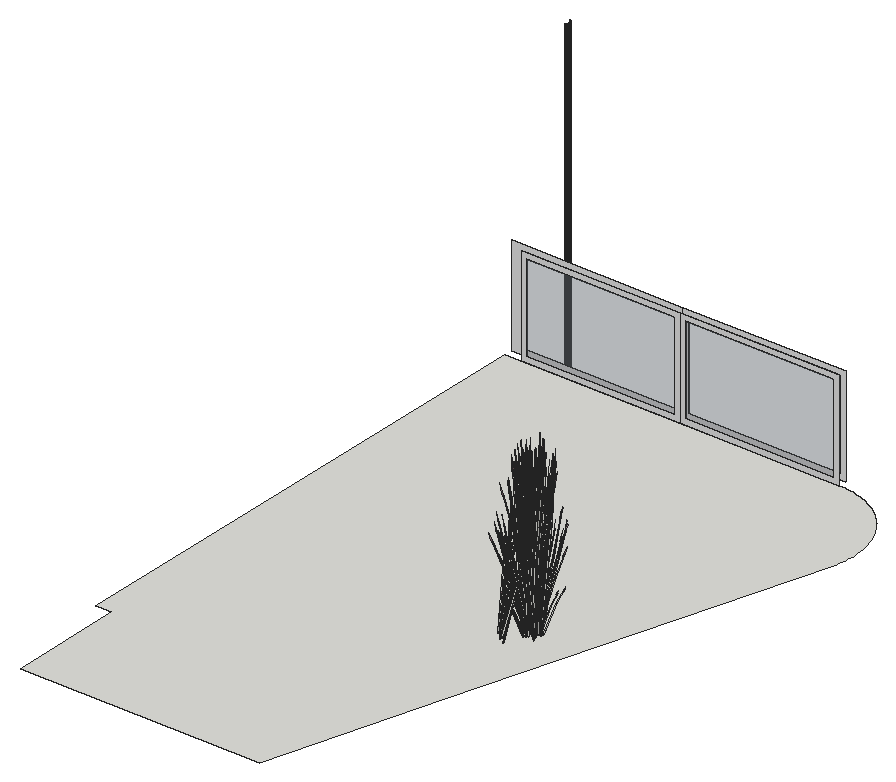
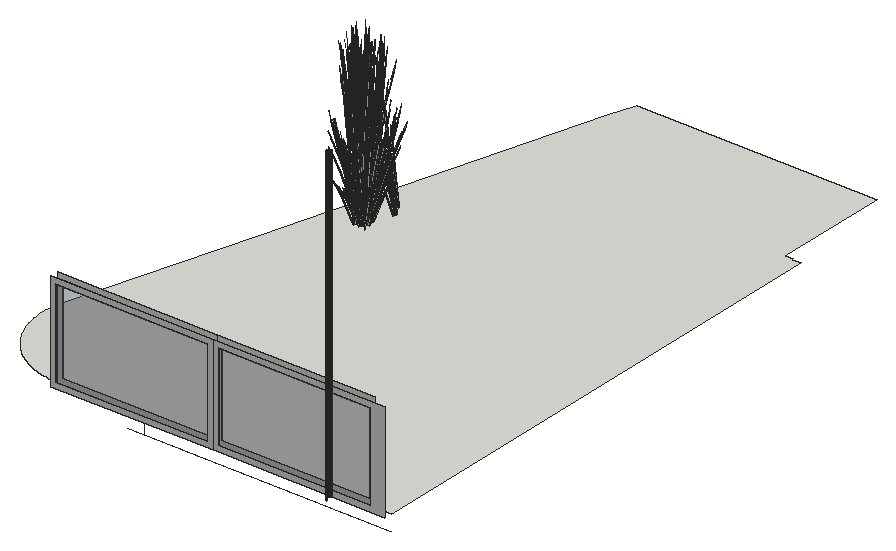
# SketchUp Ruby script. Lengths in inches.
U = 1.inch
M = Sketchup.active_model
def pt(a) = Geom::Point3d.new(a.map { |v| v * U })
def face(e, loops, mat)
  f = e.add_face(loops[0].map { |a| pt(a) })
  loops[1..].each { |l| e.add_face(l.map { |a| pt(a) }).erase! }
  f.material = f.back_material = mat if mat
  f
end
# faces: each face lists its corners as indices into pts; further lists are holes
def faces(e, pts, list, mat = nil) = list.each { |f| face(e, (f[0].is_a?(Array) ? f : [f]).map { |l| l.map { |i| pts[i] } }, mat) }
# xy, xz, yz: faces in a plane at the given z, y or x. An outline is a flat list of corners, or four numbers for a rectangle; further outlines are holes
def ring(l) = l.size == 4 ? [[l[0], l[1]], [l[2], l[1]], [l[2], l[3]], [l[0], l[3]]] : l.each_slice(2).to_a
def flat(e, list, mat, &to3) = list.each { |f| face(e, (f[0].is_a?(Array) ? f : [f]).map { |l| ring(l).map { |u, v| to3.(u, v) } }, mat) }
def xy(e, z, list, mat = nil) = flat(e, list, mat) { |x, y| [x, y, z] }
def xz(e, y, list, mat = nil) = flat(e, list, mat) { |x, z| [x, y, z] }
def yz(e, x, list, mat = nil) = flat(e, list, mat) { |y, z| [x, y, z] }
def lines(e, pts, list) = list.each { |a, b| e.add_line(pt(pts[a]), pt(pts[b])) }
# prism: a flat outline (further loops are holes) pulled along v
def prism(e, loops, v, mat = nil)
  f = face(e, loops, mat); d = Geom::Vector3d.new(v.map { |x| x * U })
  f.pushpull(f.normal.samedirection?(d) ? d.length : -d.length)
end
def box(e, o, s, mat = nil) = prism(e, [[o, [o[0] + s[0], o[1], o[2]], [o[0] + s[0], o[1] + s[1], o[2]], [o[0], o[1] + s[1], o[2]]]], [0, 0, s[2]], mat)
def at(x, y, z, deg = 0) = Geom::Transformation.translation(pt([x, y, z])) * Geom::Transformation.rotation(ORIGIN, Z_AXIS, deg.degrees)
def axes(o, x, y, z) = Geom::Transformation.new([*x, 0, *y, 0, *z, 0, *pt(o).to_a, 1])
def part(name) = M.definitions.add(name)
# library, detail: a bought-in or finely detailed component or shape, given as its bounding box
def library(name, o, s) = part(name).tap { |d| box(d.entities, o, s) }
def detail(e, o, s) = box(e.add_group.entities, o, s)
def put(e, d, t, mat = nil) = e.add_instance(d, t).tap { |i| i.material = mat if mat }
def group(e, t, mat = nil) = e.add_group.tap { |g| g.transformation = t; g.material = mat if mat }.entities
root = M.entities
M.materials.add("Glass_Basic_01").color = [105, 113, 122]
M.materials["Glass_Basic_01"].alpha = 0.25
M.materials.add("LightPink_Translucent").color = [144, 107, 117]
M.materials["LightPink_Translucent"].alpha = 0.75
M.materials.add("M01_Silver_Fog").color = [224, 224, 224]
c1 = part("blade")
p = [[2.15,0.21,22],[0,0.17,0],[0.09,0.45,0],[2.18,0.31,22],[2.29,0.31,22],[0.38,0.45,0],
  [2.48,0.24,33],[2.49,0.24,33],[2.48,0.22,33]]
faces(c1.entities,p,[[0,1,2,3],[4,5,2,3],[6,3,4,7],[8,0,3,6]])
c2 = part("seeds")
p = [[0.3,-0.1,1.38],[-0.01,-0.03,1.59],[-0.01,-0.03,0.03],[0.14,-0.07,-0.07],[0.29,-0.03,3],[0.15,0.01,3.11]]
faces(c2.entities,p,[[0,1,2,3],[1,0,4,5]],"LightPink_Translucent")
c3 = part("blade with seeds")
put(c3.entities,c1,at(0,0,0))
put(c3.entities,c2,axes([2.4,0.25,30.99],[1.5799,-0.05474,1.17369],[-0.12525,1.92788,0.29478],[-0.07173,-0.02425,1.56792]))
xy(root,522,[[216,246,303.26,246,306,255.36,321.22,307.35,340.07,371.78,359.17,437.01,359.4,437.91,359.63,439,359.83,440.1,359.98,441.21,360.09,442.32,360.16,443.43,360.1875,444.55,360.17,445.67,360.11,446.78,360.01,447.89,359.87,449,359.68,450.1,359.45,451.2,359.18,452.28,358.875,453.35,358.52,454.41,358.13,455.46,357.7,456.49,357.23,457.5,356.73,458.5,356.18,459.47,355.6,460.43,354.98,461.36,354.33,462.26,353.64,463.14,352.92,464,352.17,464.83,351.39,465.62,350.58,466.39,349.74,467.125,348.87,467.83,347.97,468.5,347.05,469.13,346.11,469.73,345.15,470.29,344.16,470.82,343.16,471.3,342.13,471.75,341.09,472.16,340.04,472.53,338.97,472.86,337.89,473.15,336.8,473.4,335.71,473.6,334.6,473.77,333.49,473.89,332.38,473.97,331.45,474,210,474,210,288,213,288,213,287.79,216,287.79]])
xz(root,474,[[218,524,271.49,556],[275.49,524,329.45,556]],"Glass_Basic_01")
xz(root,474,[[[216,522,273.49,558],[218,524,271.49,556]],[[273.49,522,331.45,558],[275.49,524,329.45,556]]],"M01_Silver_Fog")
xz(root,477,[[215,524,270.25,556],[274.25,524,329.5,556]],"Glass_Basic_01")
xz(root,477,[[[210,522,272.25,558],[215,524,270.25,556]],[[272.25,522,331.5,558],[274.25,524,329.5,556]]],"M01_Silver_Fog")
yz(root,229.87,[[478.39,522,478.47,635.24]],"M01_Silver_Fog")
p = [[229.03,477.14,522],[229.11,477.18,522],[229.11,477.18,635.24],[229.03,477.14,635.24],[229.18,477.22,522],[229.18,477.22,635.24],
  [229.26,477.27,522],[229.26,477.27,635.24],[229.33,477.32,522],[229.33,477.32,635.24],[229.4,477.38,522],[229.4,477.38,635.24],
  [229.46,477.4375,522],[229.46,477.4375,635.24],[229.52,477.5,522],[229.52,477.5,635.24],[229.58,477.57,522],[229.58,477.57,635.24],
  [229.63,477.64,522],[229.63,477.64,635.24],[229.67,477.72,522],[229.67,477.72,635.24],[229.72,477.79,522],[229.72,477.79,635.24],
  [229.75,477.875,522],[229.75,477.875,635.24],[229.79,477.96,522],[229.79,477.96,635.24],[229.8125,478.04,522],[229.8125,478.04,635.24],
  [229.83,478.125,522],[229.83,478.125,635.24],[229.85,478.21,522],[229.85,478.21,635.24],[229.86,478.3,522],[229.86,478.3,635.24],
  [229.87,478.39,522],[229.87,478.39,635.24],[229.87,478.47,522],[229.86,478.5625,522],[229.86,478.5625,635.24],[229.87,478.47,635.24],
  [229.85,478.65,522],[229.83,478.74,522],[229.83,478.74,635.24],[229.85,478.65,635.24],[229.81,478.82,522],[229.81,478.82,635.24],
  [229.78,478.9,522],[229.78,478.9,635.24],[229.75,478.99,522],[229.75,478.99,635.24],[229.71,479.07,522],[229.71,479.07,635.24],
  [229.67,479.14,522],[229.62,479.22,522],[229.62,479.22,635.24],[229.67,479.14,635.24],[229.57,479.29,522],[229.57,479.29,635.24],
  [229.51,479.35,522],[229.51,479.35,635.24],[229.45,479.42,522],[229.39,479.48,522],[229.39,479.48,635.24],[229.45,479.42,635.24],
  [229.32,479.53,522],[229.25,479.59,522],[229.25,479.59,635.24],[229.32,479.53,635.24],[229.18,479.63,522],[229.1,479.68,522],
  [229.1,479.68,635.24],[229.18,479.63,635.24],[229.02,479.71,522],[229.02,479.71,635.24],[300,474,516],[300,474,522],
  [210,474,516],[306,474,516]]
faces(root,p,[[0,1,2,3],[1,4,5,2],[4,6,7,5],[6,8,9,7],[8,10,11,9],[10,12,13,11],[12,14,15,13],[14,16,17,15],
  [16,18,19,17],[18,20,21,19],[20,22,23,21],[22,24,25,23],[24,26,27,25],[26,28,29,27],[28,30,31,29],[30,32,33,31],
  [32,34,35,33],[34,36,37,35],[38,39,40,41],[42,43,44,45],[39,42,45,40],[43,46,47,44],[46,48,49,47],[48,50,51,49],
  [50,52,53,51],[54,55,56,57],[52,54,57,53],[55,58,59,56],[58,60,61,59],[62,63,64,65],[60,62,65,61],[66,67,68,69],
  [63,66,69,64],[70,71,72,73],[67,70,73,68],[71,74,75,72]],"M01_Silver_Fog")
lines(root,p,[[76,77],[76,78],[76,79]])
put(root,c3,axes([317.24,349.05,525.875],[0.20841,-0.0122,1.71376],[-0.13825,0.52864,0.13857],[-0.297,-0.0327,0.73262]))
put(root,c3,axes([314.15,341.54,524.59],[0.15856,-0.08496,1.43002],[0.39147,0.25616,-0.30754],[-0.11652,0.22165,0.61141]))
put(root,c3,axes([317.33,349.98,525.875],[0.17434,-0.11391,1.71376],[0.14677,0.52637,0.13857],[-0.27369,0.11897,0.73262]))
put(root,c3,axes([316.79,350.875,524.59],[0.17462,0.04421,1.43002],[0.11254,0.45156,-0.30754],[-0.23719,0.08453,0.61141]))
put(root,c3,axes([314.3125,340.72,526.53],[-0.33997,0.28354,-0.35414],[-0.32182,-0.32376,0.4572],[-0.04897,0.1645,0.87481]))
put(root,c3,axes([318.33,349.43,525.34],[0.14282,-0.0779,1.77064],[0.04925,0.54394,0.13857],[-0.30935,0.07218,0.63284]))
put(root,c3,axes([317.87,348.56,526.98],[-0.50227,-0.01297,-0.71045],[0.03373,-0.54602,0.08574],[-0.21278,-0.05762,1.00501]))
put(root,c3,axes([314.54,340.42,527.34],[-0.01307,0.49815,-0.7886],[-0.55054,-0.03346,0.09517],[-0.0581,0.21104,1.11556]))
put(root,c3,axes([317.46,348.69,524.59],[0.0981,0.14994,1.43002],[-0.22605,0.40756,-0.30754],[-0.23211,-0.09741,0.61141]))
put(root,c3,axes([314.53,341.82,524.77],[-0.013,-0.32022,1.1486],[0.32493,0.22839,0.84392],[-0.0639,0.15263,0.25299]))
put(root,c3,axes([317.0625,349.5,526.53],[-0.41757,-0.15024,-0.35414],[0.12179,-0.4383,0.4572],[-0.16812,0.04019,0.87481]))
put(root,c3,axes([317.64,348.2,525.875],[0.18664,0.09279,1.71376],[-0.38624,0.38925,0.13857],[-0.24072,-0.1756,0.73262]))
put(root,c3,axes([317.35,349.73,526.68],[-0.13612,0.48987,-0.51099],[-0.46669,-0.16791,-0.3958],[-0.1879,0.04492,0.97773]))
put(root,c3,axes([314.35,341.12,525.36],[0.01104,-0.27801,1.54345],[0.49652,0.14685,0.21329],[-0.04302,0.2963,0.72882]))
put(root,c3,axes([317.7,348.67,526.68],[-0.36484,0.35674,-0.51099],[-0.31952,-0.37685,-0.3958],[-0.18537,-0.05428,0.97773]))
put(root,c3,axes([317.11,349.7,523.49],[0.01274,0.08487,1.76342],[-0.25688,0.44323,-0.26939],[-0.18246,-0.02234,0.30037]))
put(root,c3,axes([316.42,351.82,524.77],[0.2094,-0.24408,1.1486],[0.08263,0.38639,0.84392],[-0.15132,0.06919,0.25299]))
put(root,c3,axes([314.65,340.59,527],[0.35968,0.36185,-0.5672],[-0.37996,0.3169,-0.43934],[-0.05473,0.18385,1.08528]))
put(root,c3,axes([317.57,348.33,526.53],[-0.28589,-0.33718,-0.35414],[0.32644,-0.31919,0.4572],[-0.16586,-0.04856,0.87481]))
put(root,c3,axes([317.97,350.33,525.875],[0.1255,-0.16547,1.71376],[0.31687,0.44665,0.13857],[-0.21734,0.2034,0.73262]))
put(root,c3,axes([317.21,350.77,526.53],[-0.43736,0.07697,-0.35414],[-0.11549,-0.43998,0.4572],[-0.12533,0.11818,0.87481]))
put(root,c3,axes([316.98,352.07,523.49],[0.0674,0.0538,1.76342],[0.11428,0.49852,-0.26939],[-0.14937,0.10631,0.30037]))
put(root,c3,axes([314.26,341.13,524.82],[0.45645,-0.09537,0.06507],[0.10494,0.38421,-0.86304],[-0.02894,0.19449,0.7736]))
put(root,c3,axes([316.88,349.14,524.77],[0.32078,-0.03854,1.1486],[-0.20348,0.33954,0.84392],[-0.15852,-0.05093,0.25299]))
put(root,c3,axes([315.06,340.07,525.875],[-0.0123,-0.2067,1.71376],[0.53301,0.13712,0.13857],[-0.03297,0.29456,0.73262]))
put(root,c3,axes([317.875,350.74,525.875],[0.09355,-0.18511,1.71376],[0.39247,0.38307,0.13857],[-0.17705,0.23875,0.73262]))
put(root,c3,axes([317.57,350.82,526.68],[0.12908,0.49174,-0.51099],[-0.48882,0.08602,-0.3958],[-0.14008,0.13208,0.97773]))
put(root,c3,axes([318.79,350.47,524.06],[-0.52267,-0.08829,-0.62353],[0.11029,-0.54463,-0.16365],[-0.15598,-0.06599,1.37633]))
put(root,c3,axes([318.74,347.91,526.98],[-0.42844,-0.2603,-0.71045],[0.30448,-0.45614,0.08574],[-0.15523,-0.15542,1.00501]))
put(root,c3,axes([318.54,347.93,526.68],[-0.4958,0.12802,-0.51099],[-0.08673,-0.48481,-0.3958],[-0.13317,-0.13893,0.97773]))
put(root,c3,axes([318.11,351.5,524.02],[-0.47024,-0.26927,-0.49651],[0.28107,-0.48284,0],[-0.1071,-0.06133,1.57504]))
put(root,c3,axes([317.9,347.49,523.49],[-0.04867,0.07094,1.76342],[-0.49185,0.15296,-0.26939],[-0.11882,-0.13915,0.30037]))
put(root,c3,axes([318.39,351.82,524.375],[-0.31414,0.53965,0],[-0.52557,-0.30095,-0.51607],[-0.1197,-0.06854,1.63711]))
put(root,c3,axes([315.38,341.06,523.49],[0.08132,-0.0293,1.76342],[0.48914,0.1613,-0.26939],[0.0143,0.18179,0.30037]))
put(root,c3,axes([315.49,341.22,526.53],[-0.15148,0.41415,-0.35414],[-0.44193,-0.12079,0.4572],[0.04052,0.16674,0.87481]))
put(root,c3,axes([317.82,352.6,524.59],[0.15856,-0.08496,1.43002],[0.39147,0.25616,-0.30754],[-0.11652,0.22165,0.61141]))
put(root,c3,axes([317.6,347.76,524.13],[-0.14494,0.43975,-0.03893],[-0.4461,-0.13527,-0.17649],[-0.06773,-0.07192,0.58215]))
put(root,c3,axes([319.39,350.55,524.67],[-0.5073,0.35754,-0.29095],[-0.33735,-0.5052,-0.50002],[-0.12516,-0.05131,1.59708]))
put(root,c3,axes([318.59,347.57,526.53],[-0.0776,-0.43378,-0.35414],[0.44361,-0.11454,0.4572],[-0.11915,-0.12431,0.87481]))
put(root,c3,axes([317.36,349.77,524.375],[-0.62828,0,0],[0,-0.6019,-0.51607],[0,-0.13709,1.63711]))
put(root,c3,axes([318.24,351.3,524.03],[-0.11803,-0.46926,-0.30978],[0.46876,-0.13325,0.30978],[-0.0945,-0.05411,1.38974]))
put(root,c3,axes([317.98,351.79,526.53],[-0.33997,0.28354,-0.35414],[-0.32182,-0.32376,0.4572],[-0.04897,0.1645,0.87481]))
put(root,c3,axes([319.72,350.9375,524.06],[-0.33843,0.40479,-0.62353],[-0.42041,-0.36705,-0.16365],[-0.13561,0.10098,1.37633]))
put(root,c3,axes([317.84,349.61,524.33],[-0.46736,0.45277,0.30756],[-0.46764,-0.44801,-0.36492],[-0.01632,-0.12858,1.64885]))
put(root,c3,axes([315.54,340.85,526.98],[0.23981,0.43789,-0.71045],[-0.49365,0.24404,0.08574],[0.05608,0.21158,1.00501]))
put(root,c3,axes([319.77,350.86,525.33],[0.4342,0.21716,1.51261],[-0.42537,0.46784,0.59816],[-0.19053,-0.27728,1.26806]))
put(root,c3,axes([318.11,346.92,524.77],[0.2621,0.18744,1.1486],[-0.38171,0.11267,0.84392],[-0.08167,-0.14405,0.25299]))
put(root,c3,axes([319.96,350.71,524.46],[-0.49063,-0.43346,-0.25192],[0.41285,-0.48673,0.5513],[-0.13212,0.05071,1.68216]))
put(root,c3,axes([319.06,350.29,524.21],[-0.30184,-0.45202,-0.44739],[0.45719,-0.31831,0.21531],[-0.09768,-0.05593,1.43643]))
put(root,c3,axes([318.21,351.49,527.34],[-0.01307,0.49815,-0.7886],[-0.55054,-0.03346,0.09517],[-0.0581,0.21104,1.11556]))
put(root,c3,axes([318.2,352.89,524.77],[-0.013,-0.32022,1.1486],[0.32493,0.22839,0.84392],[-0.0639,0.15263,0.25299]))
put(root,c3,axes([319.71,350.62,524.21],[-0.54562,0.03324,-0.44739],[-0.04934,-0.55185,0.21531],[-0.09768,0.05593,1.43643]))
put(root,c3,axes([315.72,340.9375,526.68],[0.49392,0.135,-0.51099],[-0.1693,0.46287,-0.3958],[0.04529,0.18636,0.97773]))
put(root,c3,axes([318.66,351.54,524.48],[0.47024,0.26927,0.49651],[-0.28107,0.48284,0],[-0.1071,-0.06133,1.57504]))
put(root,c3,axes([318.03,352.1875,525.36],[0.01104,-0.27801,1.54345],[0.49652,0.14685,0.21329],[-0.04302,0.2963,0.72882]))
put(root,c3,axes([319.11,350.55,524.4375],[0.13317,-0.63814,-0.23429],[0.63143,0.11124,0.51271],[-0.11033,-0.08813,1.5644]))
put(root,c3,axes([319.34,350.7,524.62],[-0.09693,0.48062,0.1448],[-0.47357,-0.08343,-0.41347],[-0.08619,-0.04935,1.26744]))
put(root,c3,axes([320.28,352.04,524.02],[-0.47024,0.26927,-0.49651],[-0.28107,-0.48284,0],[-0.1071,0.06133,1.57504]))
put(root,c3,axes([317.5,349.36,524.02],[0,-0.53854,-0.49651],[0.56215,0,0],[0,-0.12266,1.57504]))
put(root,c3,axes([317.74,349.86,524.48],[0,0.53854,0.49651],[-0.56215,0,0],[0,-0.12266,1.57504]))
put(root,c3,axes([320.3125,351.9,524.19],[-0.31023,-0.54153,-0.05142],[0.52557,-0.30095,0.51607],[-0.12951,0.05156,1.6363]))
put(root,c3,axes([318.32,351.65,527],[0.35968,0.36185,-0.5672],[-0.37996,0.3169,-0.43934],[-0.05473,0.18385,1.08528]))
put(root,c3,axes([320.17,351.83,524.03],[-0.46876,-0.13325,-0.30978],[0.11803,-0.46926,0.30978],[-0.0945,0.05411,1.38974]))
put(root,c3,axes([318.97,349.98,524.67],[-0.56585,-0.25696,-0.29095],[0.27246,-0.54236,-0.50002],[-0.01778,-0.13316,1.59708]))
put(root,c3,axes([320.44,349.82,524.84],[-0.01373,-0.50706,1.41272],[0.62119,0.13144,0.59816],[-0.14692,0.27746,1.3335]))
put(root,c3,axes([317.93,352.2,524.82],[0.45645,-0.09537,0.06507],[0.10494,0.38421,-0.86304],[-0.02894,0.19449,0.7736]))
put(root,c3,axes([320.09,350.47,524.67],[0.05855,0.61451,-0.29095],[-0.60981,0.03716,-0.50002],[-0.10738,0.08185,1.59708]))
put(root,c3,axes([316,339.98,525.875],[-0.11485,-0.17291,1.71376],[0.53072,-0.14557,0.13857],[0.11995,0.27145,0.73262]))
put(root,c3,axes([318.71,349.44,524.1],[-0.20635,-0.55225,-0.69835],[0.59439,-0.19889,-0.18329],[-0.02281,-0.18701,1.54149]))
put(root,c3,axes([319.64,347.7,526.68],[-0.49392,-0.135,-0.51099],[0.1693,-0.46287,-0.3958],[-0.04529,-0.18636,0.97773]))
put(root,c3,axes([318.73,351.13,525.875],[-0.0123,-0.2067,1.71376],[0.53301,0.13712,0.13857],[-0.03297,0.29456,0.73262]))
put(root,c3,axes([317.74,349.37,524.03],[0.35073,-0.33601,-0.30978],[0.35073,0.33601,0.30978],[0,-0.10823,1.38974]))
put(root,c3,axes([319.32,347.2,524.13],[-0.34721,0.30895,-0.03893],[-0.31814,-0.33837,-0.17649],[-0.0224,-0.09588,0.58215]))
put(root,c3,axes([319.18,350.24,524.36],[0.63506,0.11347,0.45755],[-0.12924,0.64083,0.17955],[-0.09281,-0.06188,1.58856]))
put(root,c3,axes([319.02,350.13,524.72],[-0.24378,0.48527,0.44739],[-0.50654,-0.23354,-0.21531],[0,-0.11186,1.43643]))
put(root,c3,axes([318.84,351.27,524.47],[0.53992,-0.14294,0.17642],[0.13332,0.53195,0.35086],[-0.04815,-0.07751,1.60407]))
put(root,c3,axes([319.54,351.35,524.2],[-0.50654,-0.24178,0],[0.24378,-0.50239,0],[0,0,1.62707]))
put(root,c3,axes([320.71,351.96,524.375],[0.31414,0.53965,0],[-0.52557,0.30095,-0.51607],[-0.1197,0.06854,1.63711]))
put(root,c3,axes([320.45,351.3,524.47],[0.14515,-0.53522,0.17642],[0.53115,0.15146,0.35086],[-0.09175,0.00261,1.60407]))
put(root,c3,axes([320.2,350.59,524.62],[0.37121,0.32357,0.1448],[-0.30963,0.36505,-0.41347],[-0.08619,0.04935,1.26744]))
put(root,c3,axes([320.07,350.1875,524.3],[-0.46736,-0.46353,-0.06131],[0.46764,-0.46381,0],[-0.01632,-0.01619,1.75571]))
put(root,c3,axes([320.19,350.35,524.72],[0.54562,-0.03324,0.44739],[0.04934,0.55185,-0.21531],[-0.09768,0.05593,1.43643]))
put(root,c3,axes([320.33,351.62,524.33],[0.62903,0.17504,0.30756],[-0.15737,0.62568,-0.36492],[-0.10411,0.07831,1.64885]))
put(root,c3,axes([320.6,351.58,524.48],[0.47024,-0.26927,0.49651],[0.28107,0.48284,0],[-0.1071,0.06133,1.57504]))
put(root,c3,axes([319.13,349.65,524.36],[0.21845,0.6022,0.45755],[-0.62418,0.20941,0.17955],[0.00763,-0.11065,1.58856]))
put(root,c3,axes([319.03,349.58,524.21],[0.24378,-0.48527,-0.44739],[0.50654,0.23354,0.21531],[0,-0.11186,1.43643]))
put(root,c3,axes([319.65,351.14,524.2],[-0.16394,-0.4643,0],[0.46814,-0.1626,0],[0,0,1.54371]))
put(root,c3,axes([319.06,352.12,523.49],[0.08132,-0.0293,1.76342],[0.48914,0.1613,-0.26939],[0.0143,0.18179,0.30037]))
put(root,c3,axes([319.16,352.29,526.53],[-0.15148,0.41415,-0.35414],[-0.44193,-0.12079,0.4572],[0.04052,0.16674,0.87481]))
put(root,c3,axes([320.3125,350.23,524.21],[-0.24378,0.48527,-0.44739],[-0.50654,-0.23354,0.21531],[0,0.11186,1.43643]))
put(root,c3,axes([321.28,349.93,524.47],[-0.39477,-0.39228,0.17642],[0.39783,-0.38049,0.35086],[-0.0436,0.08011,1.60407]))
put(root,c3,axes([319.91,349.71,524.21],[0,-0.62313,0],[0.62828,0,0],[0,0,1.79456]))
put(root,c3,axes([319.33,349.82,524.43],[0.56613,0.26102,0.24065],[-0.27246,0.54236,0.50002],[0,-0.12502,1.60543]))
put(root,c3,axes([320.23,349.95,524.29],[0,0.62282,-0.05637],[-0.62828,0,0],[0,0.01957,1.79368]))
put(root,c3,axes([319.15,349.46,524.72],[-0.54562,0.03324,0.44739],[-0.04934,-0.55185,-0.21531],[0.09768,-0.05593,1.43643]))
put(root,c3,axes([318.89,348.51,524.47],[-0.14515,0.53522,0.17642],[-0.53115,-0.15146,0.35086],[0.09175,-0.00261,1.60407]))
put(root,c3,axes([319.93,351.16,524.29],[0.21845,0.61869,-0.06012],[-0.62418,0.21679,0],[0.00763,0.02161,1.72173]))
put(root,c3,axes([318.63,347.85,524.375],[-0.31414,-0.53965,0],[0.52557,-0.30095,-0.51607],[0.1197,-0.06854,1.63711]))
put(root,c3,axes([319.21,351.91,526.98],[0.23981,0.43789,-0.71045],[-0.49365,0.24404,0.08574],[0.05608,0.21158,1.00501]))
put(root,c3,axes([321.73,350.35,524.2],[-0.62797,-0.00431,-0.04976],[0,-0.6019,0.49943],[-0.01973,0.13702,1.58352]))
put(root,c3,axes([320.5,348.54,524.47],[-0.53992,0.14294,0.17642],[-0.13332,-0.53195,0.35086],[0.04815,0.07751,1.60407]))
put(root,c3,axes([319.95,346.54,524.77],[0.06446,0.31404,1.1486],[-0.35756,-0.17393,0.84392],[0.03848,-0.1608,0.25299]))
put(root,c3,axes([319.61,349.3125,524.36],[-0.4166,0.48873,0.45755],[-0.49494,-0.43142,0.17955],[0.10044,-0.04877,1.58856]))
put(root,c3,axes([320.33,350.08,524.21],[0.35073,0.34786,0],[-0.35073,0.34786,0],[0,0,1.69266]))
put(root,c3,axes([320.32,349.68,524.72],[0.24378,-0.48527,0.44739],[0.50654,0.23354,-0.21531],[0,0.11186,1.43643]))
put(root,c3,axes([320.11,351.36,524.2],[0.50654,0.24178,0],[-0.24378,0.50239,0],[0,0,1.74954]))
put(root,c3,axes([319.39,352,526.68],[0.49392,0.135,-0.51099],[-0.1693,0.46287,-0.3958],[0.04529,0.18636,0.97773]))
put(root,c3,axes([320.16,349.5625,524.38],[-0.63506,-0.11347,0.49198],[0.12924,-0.64083,0.19306],[0.09281,0.06188,1.70813]))
put(root,c3,axes([321.6,350.44,524.03],[-0.35073,0.33601,-0.30978],[-0.35073,-0.33601,0.30978],[0,0.10823,1.38974]))
put(root,c3,axes([320.6,350.375,524.09],[0.18424,0.49308,-0.69212],[-0.53071,0.17758,-0.18165],[0.02036,0.16697,1.52773]))
put(root,c3,axes([320.34,349.84,524.21],[0.56215,0,0],[0,0.55754,0],[0,0,1.78407]))
put(root,c3,axes([319.8,349.23,524.72],[-0.30184,-0.45202,0.44739],[0.45719,-0.31831,-0.21531],[0.09768,0.05593,1.43643]))
put(root,c3,axes([319.25,349.34,524.67],[-0.05855,-0.61451,-0.29095],[0.60981,-0.03716,-0.50002],[0.10738,-0.08185,1.59708]))
put(root,c3,axes([320.53,349.79,524.62],[0.46814,-0.15705,0.1448],[0.16394,0.44848,-0.41347],[0,0.0987,1.26744]))
put(root,c3,axes([320.71,348.05,526.68],[-0.35968,-0.36185,-0.51099],[0.37996,-0.3169,-0.3958],[0.05473,-0.18385,0.97773]))
put(root,c3,axes([320.375,349.82,524.67],[0.56585,0.25696,-0.29095],[-0.27246,0.54236,-0.50002],[0.01778,0.13316,1.59708]))
put(root,c3,axes([319.17,347.98,524.03],[0.46876,0.13325,-0.30978],[-0.11803,0.46926,0.30978],[0.0945,-0.05411,1.38974]))
put(root,c3,axes([321.6,349.95,524.48],[0,-0.53854,0.49651],[0.56215,0,0],[0,0.12266,1.57504]))
put(root,c3,axes([321.84,350.45,524.02],[0,0.53854,-0.49651],[-0.56215,0,0],[0,0.12266,1.57504]))
put(root,c3,axes([319.06,347.76,524.02],[0.47024,-0.26927,-0.49651],[0.28107,0.48284,0],[0.1071,-0.06133,1.57504]))
put(root,c3,axes([319.67,351.05,525.875],[-0.11485,-0.17291,1.71376],[0.53072,-0.14557,0.13857],[0.11995,0.27145,0.73262]))
put(root,c3,axes([320,349.1,524.62],[0.09693,-0.48062,0.1448],[0.47357,0.08343,-0.41347],[0.08619,0.04935,1.26744]))
put(root,c3,axes([320.67,348.27,524.48],[-0.47024,-0.26927,0.49651],[0.28107,-0.48284,0],[0.1071,0.06133,1.57504]))
put(root,c3,axes([320.26,351.08,524.18],[0.5275,-0.18273,-0.19198],[0.18536,0.52636,0.00008],[0.05823,-0.0202,1.73897]))
put(root,c3,axes([320.27,349.51,524.21],[0.30184,0.45202,-0.44739],[-0.45719,0.31831,0.21531],[0.09768,0.05593,1.43643]))
put(root,c3,axes([321.05,347.92,526.53],[0.33997,-0.28354,-0.35414],[0.32182,0.32376,0.4572],[0.04897,-0.1645,0.87481]))
put(root,c3,axes([321.13,351.5625,524.77],[-0.2829,-0.15485,1.1486],[0.36529,-0.15734,0.84392],[0.09853,0.13328,0.25299]))
put(root,c3,axes([320.12,351.4,524.59],[0.00887,-0.17852,1.43002],[0.42372,-0.19941,-0.30754],[0.1308,0.21367,0.61141]))
put(root,c3,axes([319.62,348.87,524.06],[0.33843,-0.40479,-0.62353],[0.42041,0.36705,-0.16365],[0.13561,-0.10098,1.37633]))
put(root,c3,axes([321.1,348.51,524.03],[0.11803,0.46926,-0.30978],[-0.46876,0.13325,0.30978],[0.0945,0.05411,1.38974]))
put(root,c3,axes([321.98,350.04,524.375],[0.62828,0,0],[0,0.6019,-0.51607],[0,0.13709,1.63711]))
put(root,c3,axes([319.95,349.26,524.67],[0.5073,-0.35754,-0.29095],[0.33735,0.5052,-0.50002],[0.12516,0.05131,1.59708]))
put(root,c3,axes([321.17,352.27,524.67],[-0.3222,-0.01689,1.0506],[0.21278,-0.35872,0.58006],[0.12729,0.12745,0.8241]))
put(root,c3,axes([318.67,348.94,523.59],[-0.49456,0.21561,1.28929],[-0.15741,-0.61865,0.50096],[0.30369,0.01029,1.46642]))
put(root,c3,axes([320.49,351.78,526.68],[0.4958,-0.12802,-0.51099],[0.08673,0.48481,-0.3958],[0.13317,0.13893,0.97773]))
put(root,c3,axes([320.95,347.98,524.375],[0.31414,-0.53965,0],[0.52557,0.30095,-0.51607],[0.1197,0.06854,1.63711]))
put(root,c3,axes([321.47,347.75,523.49],[-0.0752,-0.04243,1.76342],[-0.19317,-0.47398,-0.26939],[0.13031,-0.12863,0.30037]))
put(root,c3,axes([321.23,348.31,524.02],[0.47024,0.26927,-0.49651],[-0.28107,0.48284,0],[0.1071,0.06133,1.57504]))
put(root,c3,axes([321.21,352.14,523.49],[0.03661,-0.07775,1.76342],[0.46087,-0.22898,-0.26939],[0.13972,0.11851,0.30037]))
put(root,c3,axes([321.46,348.89,526.68],[-0.12908,-0.49174,-0.51099],[0.48882,-0.08602,-0.3958],[0.14008,-0.13208,0.97773]))
